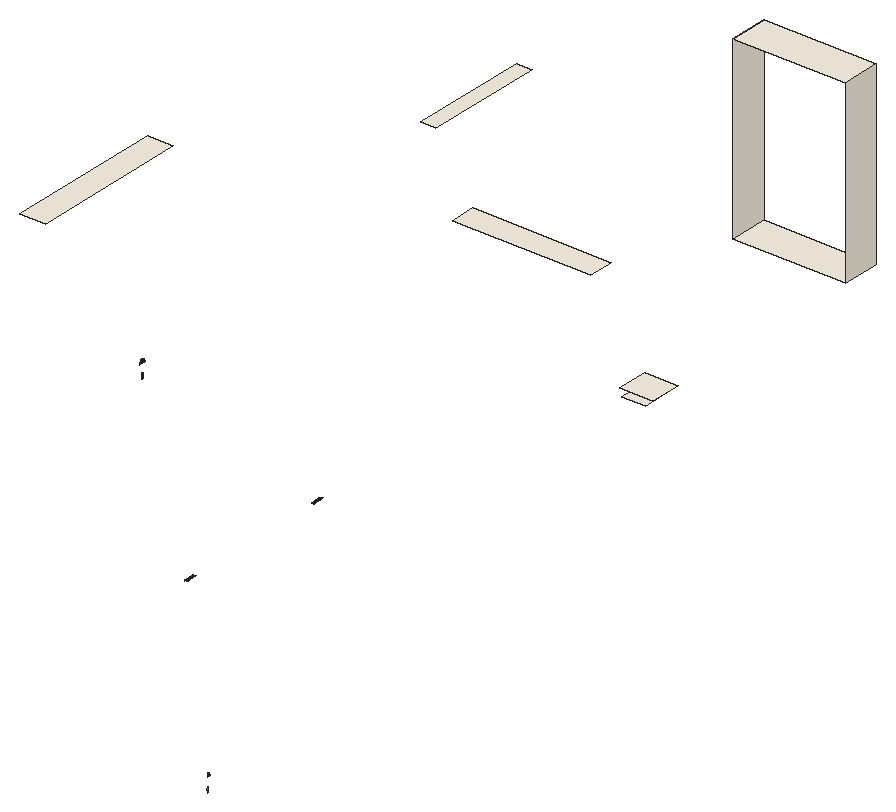
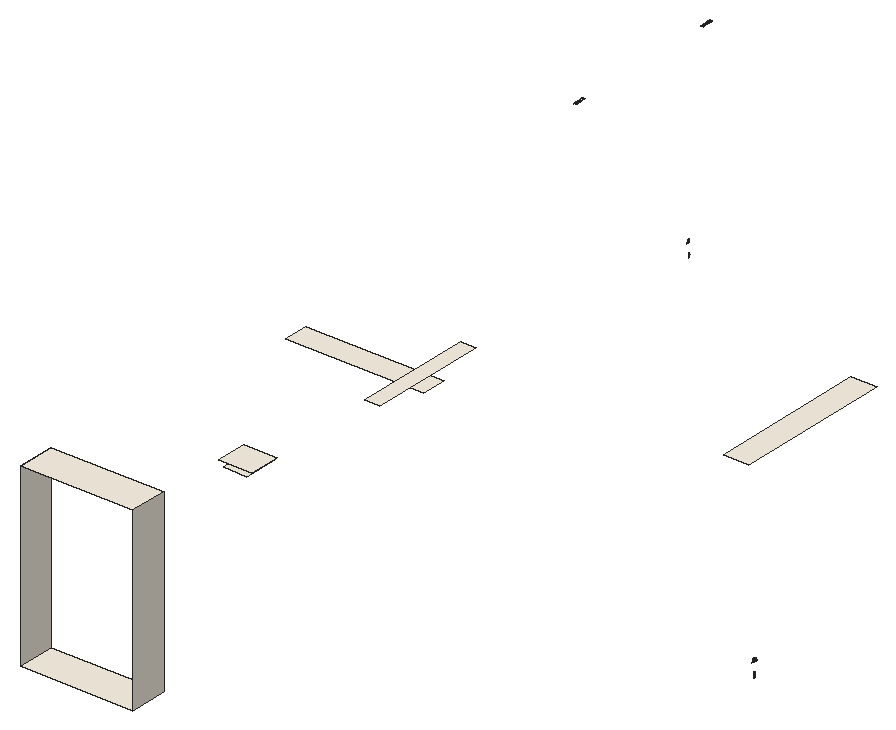
# SketchUp Ruby script. Lengths in inches.
U = 1.inch
M = Sketchup.active_model
def pt(a) = Geom::Point3d.new(a.map { |v| v * U })
def face(e, loops, mat)
  f = e.add_face(loops[0].map { |a| pt(a) })
  loops[1..].each { |l| e.add_face(l.map { |a| pt(a) }).erase! }
  f.material = f.back_material = mat if mat
  f
end
# faces: each face lists its corners as indices into pts; further lists are holes
def faces(e, pts, list, mat = nil) = list.each { |f| face(e, (f[0].is_a?(Array) ? f : [f]).map { |l| l.map { |i| pts[i] } }, mat) }
# xy, xz, yz: faces in a plane at the given z, y or x. An outline is a flat list of corners, or four numbers for a rectangle; further outlines are holes
def ring(l) = l.size == 4 ? [[l[0], l[1]], [l[2], l[1]], [l[2], l[3]], [l[0], l[3]]] : l.each_slice(2).to_a
def flat(e, list, mat, &to3) = list.each { |f| face(e, (f[0].is_a?(Array) ? f : [f]).map { |l| ring(l).map { |u, v| to3.(u, v) } }, mat) }
def xy(e, z, list, mat = nil) = flat(e, list, mat) { |x, y| [x, y, z] }
def xz(e, y, list, mat = nil) = flat(e, list, mat) { |x, z| [x, y, z] }
def yz(e, x, list, mat = nil) = flat(e, list, mat) { |y, z| [x, y, z] }
def lines(e, pts, list) = list.each { |a, b| e.add_line(pt(pts[a]), pt(pts[b])) }
# prism: a flat outline (further loops are holes) pulled along v
def prism(e, loops, v, mat = nil)
  f = face(e, loops, mat); d = Geom::Vector3d.new(v.map { |x| x * U })
  f.pushpull(f.normal.samedirection?(d) ? d.length : -d.length)
end
def box(e, o, s, mat = nil) = prism(e, [[o, [o[0] + s[0], o[1], o[2]], [o[0] + s[0], o[1] + s[1], o[2]], [o[0], o[1] + s[1], o[2]]]], [0, 0, s[2]], mat)
def at(x, y, z, deg = 0) = Geom::Transformation.translation(pt([x, y, z])) * Geom::Transformation.rotation(ORIGIN, Z_AXIS, deg.degrees)
def axes(o, x, y, z) = Geom::Transformation.new([*x, 0, *y, 0, *z, 0, *pt(o).to_a, 1])
def part(name) = M.definitions.add(name)
# library, detail: a bought-in or finely detailed component or shape, given as its bounding box
def library(name, o, s) = part(name).tap { |d| box(d.entities, o, s) }
def detail(e, o, s) = box(e.add_group.entities, o, s)
def put(e, d, t, mat = nil) = e.add_instance(d, t).tap { |i| i.material = mat if mat }
def group(e, t, mat = nil) = e.add_group.tap { |g| g.transformation = t; g.material = mat if mat }.entities
root = M.entities
M.materials.add("Material \#0").color = [86, 53, 35]
M.materials.add("Material \#1").color = [140, 140, 140]
M.materials.add("[0030_OldLace]").color = [253, 245, 230]
c1 = part("3DGeom~17_Defintion")
yz(c1.entities,-1908.8,[[-436.03,-21.87,-436.73,-21.5,-435.91,-21.83],[436.03,-21.87,435.91,-21.83,436.73,-21.5],[-435.91,-21.83,-436.73,-21.5,-436.15,-21.125],[-435.91,-21.83,-436.15,-21.125,-435.87,-21.72],[435.91,-21.83,435.87,-21.72,436.15,-21.125],
  [435.91,-21.83,436.15,-21.125,436.73,-21.5],[-436.73,-21.5,-484.73,-21.37,-436.15,-1.11],[-471.46,-21.5,-484.73,-21.37,-436.73,-21.5],[-477.2,-21.5,-484.73,-21.37,-471.46,-21.5],[-481.82,-21.5,-484.73,-21.37,-477.2,-21.5],
  [-436.73,-21.5,-436.15,-1.11,-436.15,-21.125],[436.73,-21.5,436.15,-21.125,471.46,-21.5],[471.46,-21.5,436.15,-21.125,477.2,-21.5],[477.2,-21.5,436.15,-21.125,499.98,-0.85],[477.2,-21.5,499.98,-0.85,481.82,-21.5],
  [481.82,-21.5,487.35,-21,484.73,-21.37],[481.82,-21.5,491.8,-19.52,487.35,-21],[481.82,-21.5,497.64,-13.67,491.8,-19.52],[481.82,-21.5,499.98,-0.85,497.64,-13.67],[-484.73,-21.37,-498.5,-11.58,-499.84,-0.37],
  [-484.73,-21.37,-499.84,-0.37,-499.4,-0.5],[-484.73,-21.37,-499.4,-0.5,-436.15,-1.11],[-484.73,-21.37,-493.63,-18.42,-498.5,-11.58],[-484.73,-21.37,-489.71,-20.375,-493.63,-18.42],[-484.73,-21.37,-487.35,-21,-489.71,-20.375],
  [436.15,-21.125,436.15,-1.11,436.73,-0.74],[436.15,-21.125,436.73,-0.74,499.98,-0.85],[487.35,-21,491.8,-19.52,489.71,-20.375],[-489.71,-20.375,-491.8,-19.52,-493.63,-18.42],[491.8,-19.52,495.21,-17.08,493.63,-18.42],
  [491.8,-19.52,497.64,-13.67,495.21,-17.08],[-493.63,-18.42,-496.54,-15.5,-498.5,-11.58],[-493.63,-18.42,-495.21,-17.08,-496.54,-15.5],[495.21,-17.08,497.64,-13.67,496.54,-15.5],[-496.54,-15.5,-497.64,-13.67,-498.5,-11.58],
  [497.64,-13.67,499.125,-9.22,498.5,-11.58],[497.64,-13.67,499.625,-3.69,499.125,-9.22],[497.64,-13.67,499.98,-0.85,499.625,-3.69],[-498.5,-11.58,-499.625,-3.69,-499.84,-0.37],[-498.5,-11.58,-499.5,-6.6,-499.625,-3.69],
  [-498.5,-11.58,-499.125,-9.22,-499.5,-6.6],[499.125,-9.22,499.625,-3.69,499.5,-6.6],[-499.625,-3.69,-499.98,-0.85,-500,-0.52],[-499.625,-3.69,-500,-0.52,-499.84,-0.37],[-436.15,-1.11,-499.4,-0.5,-471.46,-0.74],
  [-436.15,-1.11,-471.46,-0.74,-436.73,-0.74],[-436.15,-1.11,-436.73,-0.74,-435.91,-0.41],[-436.15,-1.11,-435.91,-0.41,-435.87,-0.52],[436.15,-1.11,435.87,-0.52,435.91,-0.41],[436.15,-1.11,435.91,-0.41,436.73,-0.74],
  [499.98,-0.85,436.73,-0.74,471.46,-0.74],[499.98,-0.85,471.46,-0.74,499.4,-0.5],[499.98,-0.85,499.4,-0.5,499.96,-0.41],[499.98,-0.85,499.96,-0.41,500,-0.52],[-436.73,-0.74,-436.03,-0.37,-435.91,-0.41],
  [436.73,-0.74,435.91,-0.41,436.03,-0.37],[-500,-0.52,-499.96,-0.41,-499.84,-0.37],[499.4,-0.5,499.84,-0.37,499.96,-0.41],[-499.84,141.21,-499.96,141.25,-499.4,141.35],[-436.03,141.21,-436.73,141.59,-435.91,141.25],
  [436.03,141.21,435.91,141.25,436.73,141.59],[499.84,141.21,484.73,162.21,498.5,152.42],[499.84,141.21,499.4,141.35,484.73,162.21],[499.84,141.21,498.5,152.42,499.625,144.53],[499.84,141.21,499.625,144.53,500,141.37],
  [499.84,141.21,500,141.37,499.96,141.25],[-499.96,141.25,-500,141.37,-499.98,141.69],[-499.96,141.25,-499.98,141.69,-499.4,141.35],[-435.91,141.25,-436.73,141.59,-436.15,141.96],[-435.91,141.25,-436.15,141.96,-435.87,141.37],
  [435.91,141.25,435.87,141.37,436.15,141.96],[435.91,141.25,436.15,141.96,436.73,141.59],[-499.4,141.35,-499.98,141.69,-471.46,141.59],[499.4,141.35,436.15,141.96,484.73,162.21],[499.4,141.35,471.46,141.59,436.15,141.96],
  [500,141.37,499.625,144.53,499.98,141.69],[-436.73,141.59,-499.98,141.69,-436.15,161.97],[-471.46,141.59,-499.98,141.69,-436.73,141.59],[-436.73,141.59,-436.15,161.97,-436.15,141.96],[436.73,141.59,436.15,141.96,471.46,141.59],
  [-499.98,141.69,-477.2,162.34,-436.15,161.97],[-499.98,141.69,-481.82,162.34,-477.2,162.34],[-499.98,141.69,-497.64,154.51,-481.82,162.34],[-499.98,141.69,-499.625,144.53,-497.64,154.51],[436.15,141.96,436.15,161.97,436.73,162.34],
  [436.15,141.96,436.73,162.34,484.73,162.21],[-499.625,144.53,-499.125,150.07,-497.64,154.51],[-499.625,144.53,-499.5,147.44,-499.125,150.07],[499.625,144.53,498.5,152.42,499.5,147.44],[499.5,147.44,498.5,152.42,499.125,150.07],
  [-499.125,150.07,-498.5,152.42,-497.64,154.51],[498.5,152.42,484.73,162.21,493.63,159.26],[498.5,152.42,493.63,159.26,496.54,156.34],[498.5,152.42,496.54,156.34,497.64,154.51],[-497.64,154.51,-491.8,160.36,-481.82,162.34],
  [-497.64,154.51,-495.21,157.92,-491.8,160.36],[-497.64,154.51,-496.54,156.34,-495.21,157.92],[496.54,156.34,493.63,159.26,495.21,157.92],[-495.21,157.92,-493.63,159.26,-491.8,160.36],[493.63,159.26,484.73,162.21,489.71,161.22],
  [493.63,159.26,489.71,161.22,491.8,160.36],[-491.8,160.36,-487.35,161.84,-481.82,162.34],[-491.8,160.36,-489.71,161.22,-487.35,161.84],[489.71,161.22,484.73,162.21,487.35,161.84],[-487.35,161.84,-484.73,162.21,-481.82,162.34],
  [-436.15,161.97,-477.2,162.34,-471.46,162.34],[-436.15,161.97,-471.46,162.34,-436.73,162.34],[-436.15,161.97,-436.73,162.34,-435.91,162.68],[-436.15,161.97,-435.91,162.68,-435.87,162.56],[436.15,161.97,435.87,162.56,435.91,162.68],
  [436.15,161.97,435.91,162.68,436.73,162.34],[484.73,162.21,436.73,162.34,471.46,162.34],[484.73,162.21,471.46,162.34,477.2,162.34],[484.73,162.21,477.2,162.34,481.82,162.34],[-436.73,162.34,-436.03,162.72,-435.91,162.68],
  [436.73,162.34,435.91,162.68,436.03,162.72]],"Material \#0")
xy(root,57.5811,[[155.7629,443.9968,155.7629,444.049,155.7863,443.9968],[155.7863,443.9968,155.7629,444.049,155.7863,444.049]],"Material \#1")
xy(root,57.9829,[[155.7629,444.002,155.7863,444.002,155.7863,444.0333],[155.7629,444.002,155.7863,444.0333,155.7629,444.0333]],"Material \#1")
xy(root,70.875,[[223.25,535.4649,250.125,544.4649]],"[0030_OldLace]")
xy(root,78.7852,[[253.3525,464.8399,258.9562,472.9649]],"[0030_OldLace]")
xy(root,79.9408,[[252.1969,465.4649,260.1117,472.9649]],"[0030_OldLace]")
xy(root,106,[[153,411.2149,159,449.0274],[217.25,459.4649,250.125,465.4649]],"[0030_OldLace]")
xy(root,113.5625,[[223.25,535.4649,250.125,544.4649]],"[0030_OldLace]")
xy(root,120,[[204.9627,465.4649,208.5578,493.9024]],"[0030_OldLace]")
xz(root,443.9941,[[155.7629,57.7803,155.7863,57.7803,155.7863,57.8088],[155.7629,57.7803,155.7863,57.8088,155.7629,57.8088]],"Material \#1")
xz(root,443.9968,[[155.7629,57.6665,155.7863,57.7318,155.7629,57.7318]],"Material \#1")
xz(root,444.002,[[155.7629,57.8373,155.7863,57.8373,155.7863,57.8724],[155.7629,57.8373,155.7863,57.8724,155.7629,57.8724]],"Material \#1")
xz(root,444.0437,[[155.7629,57.8724,155.7629,57.9101,155.7863,57.8724]],"Material \#1")
xz(root,444.049,[[155.7629,57.5811,155.7629,57.6464,155.7863,57.5811]],"Material \#1")
yz(root,155.7805,[[444.0231,57.4806,443.9671,57.4909,444.0231,57.4908],[444.0231,57.4806,444.0231,57.4908,444.0772,57.5007],[444.0231,57.4806,444.0772,57.5007,444.0791,57.4909],[444.0231,57.4908,443.9671,57.4909,443.969,57.5007],[443.9671,57.4909,443.915,57.521,443.969,57.5007],
  [444.0791,57.4909,444.0772,57.5007,444.1277,57.5298],[444.0791,57.4909,444.1277,57.5298,444.1313,57.521],[443.969,57.5007,443.915,57.521,443.9186,57.5298],[443.915,57.521,443.8702,57.5689,443.9186,57.5298],[444.1313,57.521,444.1277,57.5298,444.171,57.5761],
  [444.1313,57.521,444.171,57.5761,444.1761,57.5689],[443.9186,57.5298,443.8702,57.5689,443.8753,57.5761],[443.8702,57.5689,443.8358,57.6313,443.8753,57.5761],[444.1761,57.5689,444.171,57.5761,444.2042,57.6364],[444.1761,57.5689,444.2042,57.6364,444.2105,57.6313],
  [443.8753,57.5761,443.8358,57.6313,443.8421,57.6364],[443.8358,57.6313,443.8142,57.704,443.8421,57.6364],[444.2105,57.6313,444.2042,57.6364,444.2251,57.7066],[444.2105,57.6313,444.2251,57.7066,444.2321,57.704],[443.8421,57.6364,443.8142,57.704,443.8212,57.7066],
  [443.8142,57.704,443.8068,57.782,443.8212,57.7066],[444.2321,57.704,444.2251,57.7066,444.2322,57.782],[444.2321,57.704,444.2322,57.782,444.2395,57.782],[443.8212,57.7066,443.8068,57.782,443.8141,57.782],[443.8068,57.782,443.8142,57.86,443.8141,57.782],
  [443.8141,57.782,443.8142,57.86,443.8212,57.8574],[444.2322,57.782,444.2251,57.8574,444.2395,57.782],[444.2395,57.782,444.2251,57.8574,444.2321,57.86],[443.8212,57.8574,443.8142,57.86,443.8358,57.9327],[443.8212,57.8574,443.8358,57.9327,443.8421,57.9276],
  [444.2251,57.8574,444.2042,57.9276,444.2321,57.86],[444.2321,57.86,444.2042,57.9276,444.2105,57.9327],[443.8421,57.9276,443.8358,57.9327,443.8702,57.9951],[443.8421,57.9276,443.8702,57.9951,443.8753,57.9879],[444.2042,57.9276,444.171,57.9879,444.2105,57.9327],
  [444.2105,57.9327,444.171,57.9879,444.1761,57.9951],[443.8753,57.9879,443.8702,57.9951,443.915,58.043],[443.8753,57.9879,443.915,58.043,443.9186,58.0342],[444.171,57.9879,444.1277,58.0342,444.1761,57.9951],[444.1761,57.9951,444.1277,58.0342,444.1313,58.043],
  [443.9186,58.0342,443.915,58.043,443.9671,58.0731],[443.9186,58.0342,443.9671,58.0731,443.969,58.0633],[444.1277,58.0342,444.0772,58.0633,444.1313,58.043],[444.1313,58.043,444.0772,58.0633,444.0791,58.0731],[443.969,58.0633,443.9671,58.0731,444.0231,58.0834],
  [443.969,58.0633,444.0231,58.0834,444.0231,58.0732],[444.0772,58.0633,444.0231,58.0732,444.0791,58.0731],[444.0791,58.0731,444.0231,58.0732,444.0231,58.0834]],"Material \#1")
yz(root,155.7831,[[443.403,60.7893,443.3922,60.79,443.4027,60.9536],[443.403,60.7893,443.4027,60.9536,443.4134,60.9509],[444.6432,60.7893,444.6328,60.9509,444.6541,60.79],[444.6541,60.79,444.6328,60.9509,444.6435,60.9536],[444.0231,60.8553,443.9857,60.86,444.0231,60.8704],
  [444.0231,60.8553,444.0231,60.8704,444.0587,60.8749],[444.0231,60.8553,444.0587,60.8749,444.0606,60.86],[443.9857,60.86,443.9501,60.8736,443.9876,60.8749],[443.9857,60.86,443.9876,60.8749,444.0231,60.8704],[444.0606,60.86,444.0587,60.8749,444.0924,60.8878],
  [444.0606,60.86,444.0924,60.8878,444.0962,60.8736],[443.9501,60.8736,443.9174,60.8953,443.9539,60.8878],[443.9501,60.8736,443.9539,60.8878,443.9876,60.8749],[444.0962,60.8736,444.0924,60.8878,444.1234,60.9083],[444.0962,60.8736,444.1234,60.9083,444.1289,60.8953],
  [443.9539,60.8878,443.9174,60.8953,443.9229,60.9083],[443.9174,60.8953,443.8882,60.9241,443.9229,60.9083],[444.1289,60.8953,444.1234,60.9083,444.1511,60.9356],[444.1289,60.8953,444.1511,60.9356,444.1581,60.9241],[443.9229,60.9083,443.8882,60.9241,443.8952,60.9356],
  [443.8882,60.9241,443.863,60.9592,443.8952,60.9356],[444.1581,60.9241,444.1511,60.9356,444.175,60.9689],[444.1581,60.9241,444.175,60.9689,444.1833,60.9592],[443.8952,60.9356,443.863,60.9592,443.8713,60.9689],[443.4134,60.9509,443.4027,60.9536,443.432,61.102],
  [443.4134,60.9509,443.432,61.102,443.4422,61.0967],[444.6328,60.9509,444.6041,61.0967,444.6435,60.9536],[444.6435,60.9536,444.6041,61.0967,444.6142,61.102],[443.863,60.9592,443.8423,60.9999,443.8713,60.9689],[444.1833,60.9592,444.175,60.9689,444.1946,61.0075],
  [444.1833,60.9592,444.1946,61.0075,444.204,60.9999],[443.8713,60.9689,443.8423,60.9999,443.8517,61.0075],[443.8423,60.9999,443.8268,61.0455,443.8517,61.0075],[444.204,60.9999,444.1946,61.0075,444.2093,61.0507],[444.204,60.9999,444.2093,61.0507,444.2195,61.0455],
  [443.8517,61.0075,443.8268,61.0455,443.8369,61.0507],[443.8268,61.0455,443.817,61.095,443.8369,61.0507],[444.2195,61.0455,444.2093,61.0507,444.2186,61.0977],[444.2195,61.0455,444.2186,61.0977,444.2293,61.0951],[443.8369,61.0507,443.817,61.095,443.8277,61.0977],
  [443.817,61.095,443.8136,61.1472,443.8277,61.0977],[444.2293,61.0951,444.2186,61.0977,444.2218,61.1522],[444.2293,61.0951,444.2218,61.1522,444.2326,61.1523],[443.4422,61.0967,443.432,61.102,443.4787,61.2387],[443.4422,61.0967,443.4787,61.2387,443.488,61.2311],
  [444.6041,61.0967,444.5551,61.2386,444.6142,61.102],[443.8277,61.0977,443.8136,61.1472,443.8245,61.1472],[444.6142,61.102,444.5551,61.2386,444.5644,61.2463],[443.8136,61.1472,443.817,61.1994,443.8245,61.1472],[443.8245,61.1472,443.817,61.1994,443.8277,61.1967],
  [444.2218,61.1522,444.2186,61.1967,444.2326,61.1523],[444.2326,61.1523,444.2186,61.1967,444.2293,61.1995],[443.8277,61.1967,443.817,61.1994,443.8268,61.2489],[443.8277,61.1967,443.8268,61.2489,443.8369,61.2437],[444.2186,61.1967,444.2093,61.2437,444.2293,61.1995],
  [444.2293,61.1995,444.2093,61.2437,444.2195,61.2489],[443.488,61.2311,443.4787,61.2387,443.5409,61.3614],[443.488,61.2311,443.5409,61.3614,443.5492,61.3516],[444.5551,61.2386,444.4971,61.3516,444.5644,61.2463],[443.8369,61.2437,443.8268,61.2489,443.8423,61.2945],
  [443.8369,61.2437,443.8423,61.2945,443.8517,61.2869],[444.2093,61.2437,444.1946,61.2869,444.2195,61.2489],[444.5644,61.2463,444.4971,61.3516,444.5053,61.3614],[444.2195,61.2489,444.1946,61.2869,444.204,61.2945],[443.8517,61.2869,443.8423,61.2945,443.863,61.3352],
  [443.8517,61.2869,443.863,61.3352,443.8713,61.3255],[444.1946,61.2869,444.175,61.3255,444.204,61.2945],[444.204,61.2945,444.175,61.3255,444.1833,61.3352],[443.8713,61.3255,443.863,61.3352,443.8882,61.3703],[443.8713,61.3255,443.8882,61.3703,443.8952,61.3588],
  [444.175,61.3255,444.1511,61.3588,444.1833,61.3352],[444.1833,61.3352,444.1511,61.3588,444.1581,61.3703],[443.5492,61.3516,443.5409,61.3614,443.617,61.4674],[443.5492,61.3516,443.617,61.4674,443.624,61.4558],[444.4971,61.3516,444.4223,61.4558,444.5053,61.3614],
  [443.8952,61.3588,443.8882,61.3703,443.9174,61.3991],[443.8952,61.3588,443.9174,61.3991,443.9229,61.3861],[444.1511,61.3588,444.1234,61.3861,444.1581,61.3703],[444.5053,61.3614,444.4223,61.4558,444.4292,61.4674],[444.1581,61.3703,444.1234,61.3861,444.1289,61.3991],
  [443.9229,61.3861,443.9174,61.3991,443.9501,61.4208],[443.9229,61.3861,443.9501,61.4208,443.9539,61.4066],[444.1234,61.3861,444.0924,61.4066,444.1289,61.3991],[444.1289,61.3991,444.0924,61.4066,444.0962,61.4208],[443.9539,61.4066,443.9501,61.4208,443.9857,61.4344],
  [443.9539,61.4066,443.9857,61.4344,443.9876,61.4195],[444.0924,61.4066,444.0587,61.4195,444.0962,61.4208],[443.9876,61.4195,443.9857,61.4344,444.0231,61.4391],[443.9876,61.4195,444.0231,61.4391,444.0231,61.424],[444.0587,61.4195,444.0231,61.424,444.0606,61.4344],
  [444.0587,61.4195,444.0606,61.4344,444.0962,61.4208],[444.0231,61.424,444.0231,61.4391,444.0606,61.4344],[443.624,61.4558,443.617,61.4674,443.7051,61.5541],[443.624,61.4558,443.7051,61.5541,443.7105,61.5411],[444.4223,61.4558,444.3357,61.5411,444.4292,61.4674],
  [444.4292,61.4674,444.3357,61.5411,444.3412,61.5541],[443.7105,61.5411,443.7051,61.5541,443.8032,61.6191],[443.7105,61.5411,443.8032,61.6191,443.807,61.6049],[444.3357,61.5411,444.2393,61.6049,444.3412,61.5541],[444.3412,61.5541,444.2393,61.6049,444.2431,61.6191],
  [443.807,61.6049,443.8032,61.6191,443.9097,61.6599],[443.807,61.6049,443.9097,61.6599,443.9117,61.645],[444.2393,61.6049,444.1346,61.645,444.2431,61.6191],[444.2431,61.6191,444.1346,61.645,444.1365,61.6599],[443.9117,61.645,443.9097,61.6599,444.0231,61.6741],
  [443.9117,61.645,444.0231,61.6741,444.0231,61.659],[444.1346,61.645,444.0231,61.659,444.1365,61.6599],[444.0231,61.659,444.0231,61.6741,444.1365,61.6599]],"Material \#1")
yz(root,155.7856,[[444.0231,57.4405,443.8319,57.5685,443.928,57.5113],[444.0231,57.4405,443.9154,57.4752,443.8319,57.5685],[444.0231,57.4405,443.967,57.4495,443.9154,57.4752],[444.0231,57.4405,443.928,57.5113,443.9736,57.4886],[444.0231,57.4405,443.9736,57.4886,444.0231,57.4806],
  [444.0231,57.4405,444.0231,57.4806,444.0727,57.4886],[444.0231,57.4405,444.0727,57.4886,444.1182,57.5113],[444.0231,57.4405,444.1182,57.5113,444.2144,57.5685],[444.0231,57.4405,444.1309,57.4752,444.0793,57.4495],[444.0231,57.4405,444.2144,57.5685,444.1309,57.4752],
  [443.9154,57.4752,443.8698,57.5155,443.8319,57.5685],[444.1309,57.4752,444.2144,57.5685,444.1764,57.5155],[443.928,57.5113,443.8319,57.5685,443.8879,57.5469],[444.1182,57.5113,444.1584,57.5469,444.2144,57.5685],[443.8879,57.5469,443.8319,57.5685,443.8544,57.5936],
  [444.1584,57.5469,444.1919,57.5936,444.2144,57.5685],[443.8319,57.5685,443.7802,57.827,443.8288,57.6495],[443.8319,57.5685,443.7845,57.7037,443.7802,57.827],[443.8319,57.5685,443.8029,57.6319,443.7845,57.7037],[443.8319,57.5685,443.8288,57.6495,443.8544,57.5936],
  [444.2144,57.5685,444.1919,57.5936,444.2174,57.6495],[444.2144,57.5685,444.2174,57.6495,444.2337,57.7129],[444.2144,57.5685,444.2337,57.7129,444.2662,57.8272],[444.2144,57.5685,444.2618,57.7037,444.2434,57.6319],[444.2144,57.5685,444.2662,57.8272,444.2618,57.7037],
  [443.8288,57.6495,443.7802,57.827,443.8125,57.7129],[443.7845,57.7037,443.778,57.782,443.7802,57.827],[444.2618,57.7037,444.2662,57.8272,444.2683,57.782],[443.8125,57.7129,443.7802,57.827,443.8068,57.782],[444.2337,57.7129,444.2395,57.782,444.2662,57.8272],
  [443.8068,57.782,443.7802,57.827,443.8125,57.851],[444.2395,57.782,444.2337,57.851,444.2662,57.8272],[443.7802,57.827,443.7866,57.87,443.7969,57.9109],[443.7802,57.827,443.7969,57.9109,443.8276,57.985],[443.7802,57.827,443.8276,57.985,443.8738,58.0531],
  [443.7802,57.827,443.8288,57.9145,443.8125,57.851],[443.7802,57.827,443.8738,58.0531,443.8775,58.059],[443.7802,57.827,443.8775,58.059,443.8806,58.0652],[443.7802,57.827,443.8806,58.0652,443.8288,57.9145],[444.2662,57.8272,443.9163,58.5794,444.1654,58.0658],
  [444.2662,57.8272,444.1919,57.9704,443.9163,58.5794],[444.2662,57.8272,444.1654,58.0658,444.1685,58.0593],[444.2662,57.8272,444.1685,58.0593,444.1723,58.0531],[444.2662,57.8272,444.1723,58.0531,444.2195,57.9862],[444.2662,57.8272,444.2174,57.9145,444.1919,57.9704],
  [444.2662,57.8272,444.2337,57.851,444.2174,57.9145],[444.2662,57.8272,444.2195,57.9862,444.2499,57.9118],[444.2662,57.8272,444.2499,57.9118,444.2599,57.8706],[443.7969,57.9109,443.8107,57.9493,443.8276,57.985],[444.2499,57.9118,444.2195,57.9862,444.2363,57.9504],
  [443.8288,57.9145,443.8806,58.0652,443.8544,57.9704],[443.8544,57.9704,443.8806,58.0652,443.8847,58.0789],[443.8544,57.9704,443.8847,58.0789,443.8879,58.0171],[444.1919,57.9704,444.1584,58.0171,443.9163,58.5794],[443.8276,57.985,443.8473,58.0178,443.8694,58.0475],
  [443.8276,57.985,443.8694,58.0475,443.8738,58.0531],[444.2195,57.9862,444.1723,58.0531,444.177,58.0473],[444.2195,57.9862,444.177,58.0473,444.1996,58.0186],[443.8879,58.0171,443.8847,58.0789,443.8861,58.0949],[443.8879,58.0171,443.8861,58.0949,443.8861,58.46],
  [443.8879,58.0171,443.8861,58.46,443.928,58.0527],[444.1584,58.0171,444.1182,58.0527,443.9163,58.5794],[443.928,58.0527,443.8861,58.46,443.9736,58.0754],[444.1182,58.0527,444.0727,58.0754,443.9163,58.5794],[443.8806,58.0652,443.883,58.0718,443.8847,58.0789],
  [444.1654,58.0658,443.9163,58.5794,444.1631,58.0726],[444.1631,58.0726,443.9163,58.5794,444.1614,58.0797],[443.9736,58.0754,443.8861,58.46,444.0231,58.0834],[444.0727,58.0754,444.0231,58.0834,443.9163,58.5794],[443.8847,58.0789,443.8858,58.0866,443.8861,58.0949],
  [444.1614,58.0797,443.9163,58.5794,444.1605,58.0871],[444.0231,58.0834,443.8861,58.46,443.9163,58.5794],[444.1605,58.0871,443.9163,58.5794,444.13,58.5794],[444.1605,58.0871,444.13,58.5794,444.1601,58.0949],[444.1601,58.0949,444.13,58.5794,444.1565,58.5038],
  [444.1601,58.0949,444.1565,58.5038,444.1601,58.46],[443.8861,58.46,443.8898,58.5038,443.9163,58.5794],[443.8898,58.5038,443.9001,58.5439,443.9163,58.5794],[444.1565,58.5038,444.13,58.5794,444.1462,58.5439],[443.9163,58.5794,443.9375,58.609,443.9629,58.6315],
  [443.9163,58.5794,443.9629,58.6315,444.0231,58.6509],[443.9163,58.5794,444.0231,58.6509,444.13,58.5794],[444.13,58.5794,444.0231,58.6509,444.0834,58.6315],[444.13,58.5794,444.0834,58.6315,444.1088,58.609],[443.9629,58.6315,443.9917,58.6459,444.0231,58.6509],
  [444.0834,58.6315,444.0231,58.6509,444.0545,58.6459]],"Material \#1")
yz(root,155.7863,[[444.0231,57.5134,443.9732,57.5226,444.0231,57.5235],[444.0231,57.5134,444.0231,57.5235,444.0711,57.5323],[444.0231,57.5134,444.0711,57.5323,444.073,57.5226],[443.9732,57.5226,443.9267,57.5494,443.9751,57.5323],[443.9732,57.5226,443.9751,57.5323,444.0231,57.5235],
  [444.073,57.5226,444.0711,57.5323,444.1159,57.5582],[444.073,57.5226,444.1159,57.5582,444.1195,57.5494],[443.9751,57.5323,443.9267,57.5494,443.9304,57.5582],[443.9267,57.5494,443.8868,57.5921,443.9304,57.5582],[444.1195,57.5494,444.1159,57.5582,444.1543,57.5992],
  [444.1195,57.5494,444.1543,57.5992,444.1595,57.5921],[443.9304,57.5582,443.8868,57.5921,443.8919,57.5992],[443.8868,57.5921,443.8562,57.6477,443.8919,57.5992],[444.1595,57.5921,444.1543,57.5992,444.1838,57.6528],[444.1595,57.5921,444.1838,57.6528,444.1901,57.6477],
  [443.8919,57.5992,443.8562,57.6477,443.8625,57.6528],[443.8562,57.6477,443.8369,57.7125,443.8625,57.6528],[444.1901,57.6477,444.1838,57.6528,444.2023,57.7151],[444.1901,57.6477,444.2023,57.7151,444.2094,57.7125],[443.8625,57.6528,443.8369,57.7125,443.8439,57.7151],
  [443.8369,57.7125,443.8303,57.782,443.8439,57.7151],[444.2094,57.7125,444.2023,57.7151,444.2087,57.782],[444.2094,57.7125,444.2087,57.782,444.2159,57.782],[443.8439,57.7151,443.8303,57.782,443.8376,57.782],[443.8303,57.782,443.8369,57.8515,443.8376,57.782],
  [443.8376,57.782,443.8369,57.8515,443.8439,57.8489],[444.2087,57.782,444.2023,57.8489,444.2159,57.782],[444.2159,57.782,444.2023,57.8489,444.2094,57.8515],[443.8439,57.8489,443.8369,57.8515,443.8562,57.9163],[443.8439,57.8489,443.8562,57.9163,443.8625,57.9112],
  [444.2023,57.8489,444.1838,57.9112,444.2094,57.8515],[444.2094,57.8515,444.1838,57.9112,444.1901,57.9163],[443.8625,57.9112,443.8562,57.9163,443.8868,57.9719],[443.8625,57.9112,443.8868,57.9719,443.8919,57.9648],[444.1838,57.9112,444.1543,57.9648,444.1901,57.9163],
  [444.1901,57.9163,444.1543,57.9648,444.1595,57.9719],[443.8919,57.9648,443.8868,57.9719,443.9267,58.0146],[443.8919,57.9648,443.9267,58.0146,443.9304,58.0058],[444.1543,57.9648,444.1159,58.0058,444.1595,57.9719],[444.1595,57.9719,444.1159,58.0058,444.1195,58.0146],
  [443.9304,58.0058,443.9267,58.0146,443.9732,58.0414],[443.9304,58.0058,443.9732,58.0414,443.9751,58.0316],[444.1159,58.0058,444.0711,58.0316,444.1195,58.0146],[444.1195,58.0146,444.0711,58.0316,444.073,58.0414],[443.9751,58.0316,443.9732,58.0414,444.0231,58.0506],
  [443.9751,58.0316,444.0231,58.0506,444.0231,58.0405],[444.0711,58.0316,444.0231,58.0405,444.073,58.0414],[444.0231,58.0405,444.0231,58.0506,444.073,58.0414]],"Material \#1")
yz(root,223.25,[[535.4649,70.875,544.4649,113.5625]],"[0030_OldLace]")
yz(root,250.125,[[535.4649,70.875,544.4649,113.5625]],"[0030_OldLace]")
yz(root,263.9496,[[328.1772,58.0499,328.1772,58.0895,328.2287,58.0973],[328.1772,58.0499,328.2287,58.0973,328.2761,58.1197],[328.1772,58.0499,328.2761,58.1197,328.3761,58.1761],[328.1772,58.0499,328.2893,58.0841,328.2356,58.0588],[328.1772,58.0499,328.3761,58.1761,328.2893,58.0841],
  [328.2893,58.0841,328.3761,58.1761,328.3366,58.1239],[328.2761,58.1197,328.3178,58.1548,328.3761,58.1761],[328.3178,58.1548,328.3527,58.2009,328.3761,58.1761],[328.3761,58.1761,328.3527,58.2009,328.3793,58.256],[328.3761,58.1761,328.3793,58.256,328.4298,58.4311],
  [328.3761,58.1761,328.4254,58.3095,328.4062,58.2386],[328.3761,58.1761,328.4298,58.4311,328.4254,58.3095],[328.3793,58.256,328.3962,58.3186,328.4298,58.4311],[328.4254,58.3095,328.4298,58.4311,328.4321,58.3867],[328.3962,58.3186,328.4021,58.3867,328.4298,58.4311],
  [328.4021,58.3867,328.3962,58.4548,328.4298,58.4311],[328.4298,58.4311,328.3255,58.666,328.3287,58.6599],[328.4298,58.4311,328.3793,58.5173,328.3255,58.666],[328.4298,58.4311,328.3287,58.6599,328.3325,58.6541],[328.4298,58.4311,328.3325,58.6541,328.3805,58.5869],
  [328.4298,58.4311,328.3962,58.4548,328.3793,58.5173],[328.4298,58.4311,328.3805,58.5869,328.4125,58.5138],[328.4298,58.4311,328.4125,58.5138,328.4231,58.4735],[328.4125,58.5138,328.3805,58.5869,328.3981,58.5517],[328.3793,58.5173,328.3527,58.5725,328.3255,58.666],
  [328.3527,58.5725,328.3178,58.6185,328.3211,58.6795],[328.3527,58.5725,328.3211,58.6795,328.3255,58.666],[328.3805,58.5869,328.3325,58.6541,328.337,58.6485],[328.3805,58.5869,328.337,58.6485,328.36,58.6193],[328.3178,58.6185,328.2761,58.6536,328.3197,59.0553],
  [328.3178,58.6185,328.3197,58.6953,328.3211,58.6795],[328.3178,58.6185,328.3197,59.0553,328.3197,58.6953],[328.2761,58.6536,328.2287,58.676,328.3197,59.0553],[328.3255,58.666,328.3211,58.6795,328.3229,58.6725],[328.1257,58.676,328.2883,59.173,328.1772,58.6839],
  [328.2287,58.676,328.1772,58.6839,328.3197,59.0553],[328.3211,58.6795,328.3197,58.6953,328.32,58.687],[328.1772,58.6839,328.2883,59.173,328.3197,59.0553],[328.3197,59.0553,328.2883,59.173,328.3159,59.0985],[328.3159,59.0985,328.2883,59.173,328.3052,59.1381],
  [328.2883,59.173,328.1772,59.2436,328.2398,59.2244],[328.2883,59.173,328.2398,59.2244,328.2663,59.2022],[328.2398,59.2244,328.1772,59.2436,328.2098,59.2386]],"Material \#1")
yz(root,263.9522,[[328.8221,61.3524,328.8223,61.5144,328.8333,61.3531],[328.2162,61.4221,328.1772,61.4324,328.2141,61.4368],[328.2162,61.4221,328.2141,61.4368,328.2531,61.4356],[328.2531,61.4356,328.2141,61.4368,328.2492,61.4495],[328.2531,61.4356,328.2492,61.4495,328.2872,61.4569],
  [328.2492,61.4495,328.2815,61.4698,328.2872,61.4569],[328.2872,61.4569,328.2815,61.4698,328.3175,61.4853],[328.2815,61.4698,328.3103,61.4967,328.3175,61.4853],[328.3175,61.4853,328.3103,61.4967,328.3438,61.5199],[328.3103,61.4967,328.3351,61.5295,328.3438,61.5199],
  [328.3438,61.5199,328.3351,61.5295,328.3652,61.5601],[328.3351,61.5295,328.3555,61.5676,328.3652,61.5601],[328.3652,61.5601,328.3555,61.5676,328.3814,61.605],[328.3555,61.5676,328.3708,61.6102,328.3814,61.605],[328.3814,61.605,328.3708,61.6102,328.3916,61.6539],
  [328.3708,61.6102,328.3805,61.6565,328.3916,61.6539],[328.3916,61.6539,328.3805,61.6565,328.3951,61.7054],[328.7813,61.6556,328.7336,61.7881,328.7434,61.7956],[328.3805,61.6565,328.3838,61.7054,328.3951,61.7054],[328.3838,61.7054,328.3805,61.7542,328.3916,61.7568],
  [328.3838,61.7054,328.3916,61.7568,328.3951,61.7054],[328.3805,61.7542,328.3708,61.8005,328.3814,61.8057],[328.3805,61.7542,328.3814,61.8057,328.3916,61.7568],[328.7336,61.7881,328.67,61.907,328.6786,61.9166],[328.7336,61.7881,328.6786,61.9166,328.7434,61.7956],
  [328.3708,61.8005,328.3555,61.8431,328.3652,61.8506],[328.3708,61.8005,328.3652,61.8506,328.3814,61.8057],[328.3555,61.8431,328.3351,61.8812,328.3438,61.8908],[328.3555,61.8431,328.3438,61.8908,328.3652,61.8506],[328.3351,61.8812,328.3103,61.914,328.3175,61.9254],
  [328.3351,61.8812,328.3175,61.9254,328.3438,61.8908],[328.67,61.907,328.5922,62.0097,328.5995,62.0211],[328.67,61.907,328.5995,62.0211,328.6786,61.9166],[328.3103,61.914,328.2815,61.9409,328.2872,61.9538],[328.3103,61.914,328.2872,61.9538,328.3175,61.9254],
  [328.2815,61.9409,328.2492,61.9612,328.2531,61.9751],[328.2815,61.9409,328.2531,61.9751,328.2872,61.9538],[328.2492,61.9612,328.2141,61.9739,328.2162,61.9886],[328.2492,61.9612,328.2162,61.9886,328.2531,61.9751],[328.2141,61.9739,328.1772,61.9932,328.2162,61.9886],
  [328.5922,62.0097,328.5023,62.0938,328.508,62.1067],[328.5922,62.0097,328.508,62.1067,328.5995,62.0211],[328.5023,62.0938,328.402,62.1568,328.4059,62.1707],[328.5023,62.0938,328.4059,62.1707,328.508,62.1067],[328.402,62.1568,328.2931,62.1963,328.2951,62.211],
  [328.402,62.1568,328.2951,62.211,328.4059,62.1707],[328.2931,62.1963,328.1772,62.21,328.1772,62.225],[328.2931,62.1963,328.1772,62.225,328.2951,62.211]],"Material \#1")
p = [[155.7863,443.9996,57.6542],[155.7629,443.9968,57.6464],[155.7629,443.9968,57.5811],[155.7629,444.049,57.6464],[155.7863,444.0466,57.6608],[155.7863,444.049,57.5811],
  [155.7629,443.9968,57.5811],[155.7863,443.9968,57.5811],[155.7863,443.9996,57.6542],[155.7863,444.0463,57.7418],[155.7629,444.0437,57.7519],[155.7629,444.0517,57.7803],
  [155.7863,444.0488,57.7274],[155.7629,444.049,57.7318],[155.7629,444.0437,57.7519],[155.7863,444.0466,57.6608],[155.7629,444.049,57.6665],[155.7629,444.049,57.7318],
  [155.7863,444.002,57.7519],[155.7629,444.002,57.7519],[155.7629,443.9968,57.7318],[155.7629,444.0517,57.7803],[155.7863,444.0477,57.7661],[155.7863,444.0463,57.7418],
  [155.7629,444.0437,57.7519],[155.7863,444.0463,57.7418],[155.7863,444.0488,57.7274],[155.7629,444.049,57.7318],[155.7863,444.0488,57.7274],[155.7863,444.0466,57.6608],
  [155.7629,443.9968,57.7318],[155.7863,443.9968,57.7318],[155.7863,444.002,57.7519],[155.7629,443.9968,57.6665],[155.7863,443.9996,57.6542],[155.7863,443.9968,57.7318],
  [155.7863,444.002,57.8373],[155.7629,444.002,57.8373],[155.7629,443.9941,57.8088],[155.7863,443.9941,57.7803],[155.7629,443.9941,57.7803],[155.7629,444.002,57.7519],
  [155.7863,444.0477,57.823],[155.7629,444.0437,57.8373],[155.7629,444.0437,57.8724],[155.7863,444.0517,57.7946],[155.7629,444.0517,57.8088],[155.7629,444.0437,57.8373],
  [155.7629,443.9941,57.8088],[155.7863,443.9941,57.8088],[155.7863,444.002,57.8373],[155.7629,444.002,57.7519],[155.7863,444.002,57.7519],[155.7863,443.9941,57.7803],
  [155.7629,444.0517,57.8088],[155.7863,444.0517,57.7946],[155.7863,444.0477,57.7661],[155.7629,444.0437,57.8724],[155.7863,444.0437,57.8724],[155.7863,444.0477,57.823],
  [155.7629,444.0437,57.8373],[155.7863,444.0477,57.823],[155.7863,444.0517,57.7946],[155.7863,444.0097,57.9477],[155.7629,444.0124,57.9528],[155.7629,444.0069,57.9427],
  [155.7863,444.0097,57.9151],[155.7629,444.0069,57.9201],[155.7629,444.0124,57.9101],[155.7863,444.0097,57.9151],[155.7629,444.0124,57.9101],[155.7629,444.002,57.8724],
  [155.7863,444.0465,57.9477],[155.7629,444.0493,57.9427],[155.7629,444.0437,57.9528],[155.7863,444.0465,57.9151],[155.7629,444.0437,57.9101],[155.7629,444.0493,57.9201],
  [155.7863,444.0097,57.9477],[155.7629,444.0069,57.9427],[155.7629,444.0069,57.9201],[155.7863,444.0097,57.9151],[155.7863,444.0465,57.9151],[155.7629,444.0493,57.9201],
  [155.7629,444.0493,57.9427],[155.7863,444.0465,57.9477],[155.7629,444.0124,57.9528],[155.7863,444.0097,57.9477],[155.7863,444.002,57.9829],[155.7629,444.002,57.8724],
  [155.7863,444.002,57.8724],[155.7863,444.0097,57.9151],[155.7629,444.0437,57.9101],[155.7863,444.0465,57.9151],[155.7863,444.0437,57.8724],[155.7863,444.002,57.9829],
  [155.7629,444.002,57.9829],[155.7629,444.0124,57.9528],[155.7831,443.9508,61.0626],[155.7811,443.9508,61.0626],[155.7805,443.9349,61.0314],[155.7825,443.9349,61.0314],
  [155.7805,443.9532,61.008],[155.7825,443.9532,61.008],[155.7805,443.975,60.9922],[155.7825,443.975,60.9922],[155.7811,443.9908,61.0236],[155.7831,443.9908,61.0236],
  [155.7813,444.0049,61.0517],[155.7833,444.0049,61.0517],[155.7833,443.965,61.0906],[155.7813,443.965,61.0906],[155.7813,444.0812,61.2037],[155.7833,444.0812,61.2037],
  [155.7833,444.0415,61.2427],[155.7813,444.0415,61.2427],[155.7831,444.0554,61.2708],[155.7811,444.0554,61.2708],[155.7811,444.0955,61.2318],[155.7831,444.0955,61.2318],
  [155.7805,444.1113,61.2632],[155.7825,444.1113,61.2632],[155.7805,444.0931,61.2864],[155.7825,444.0931,61.2864],[155.7805,444.071,61.3025],[155.7825,444.071,61.3025]]
faces(root,p,[[0,1,2],[3,4,5],[6,7,8],[9,10,11],[12,13,14],[15,16,17],[18,19,20],[21,22,23],
  [24,25,26],[27,28,29],[30,31,32],[33,34,35],[36,37,38],[39,40,41],[42,43,44],[45,46,47],
  [48,49,50],[51,52,53],[54,55,56],[57,58,59],[60,61,62],[63,64,65],[66,67,68],[69,70,71],
  [72,73,74],[75,76,77],[78,79,80],[80,81,78],[82,83,84],[84,85,82],[86,87,88],[89,90,91],
  [92,93,94],[95,96,97],[98,99,100],[100,101,98],[101,100,102],[102,103,101],[103,102,104],[104,105,103],
  [105,104,106],[106,107,105],[107,106,108],[108,109,107],[110,111,99],[99,98,110],[109,108,112],[112,113,109],
  [114,115,111],[111,110,114],[116,117,115],[115,114,116],[113,112,118],[118,119,113],[119,118,120],[120,121,119],
  [121,120,122],[122,123,121],[123,122,124],[124,125,123],[125,124,117],[117,116,125]],"Material \#1")
put(root,c1,axes([263.65,342.05,3.9],[0,0,-0.05346],[0,0.04046,0],[0.00276,0,0]),"Material \#0")
